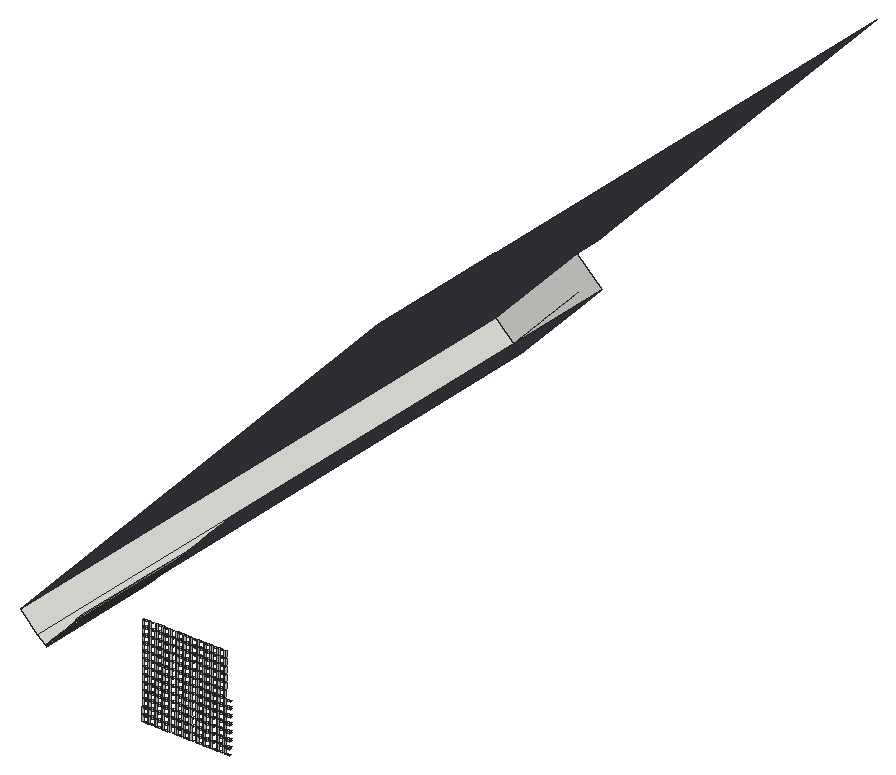
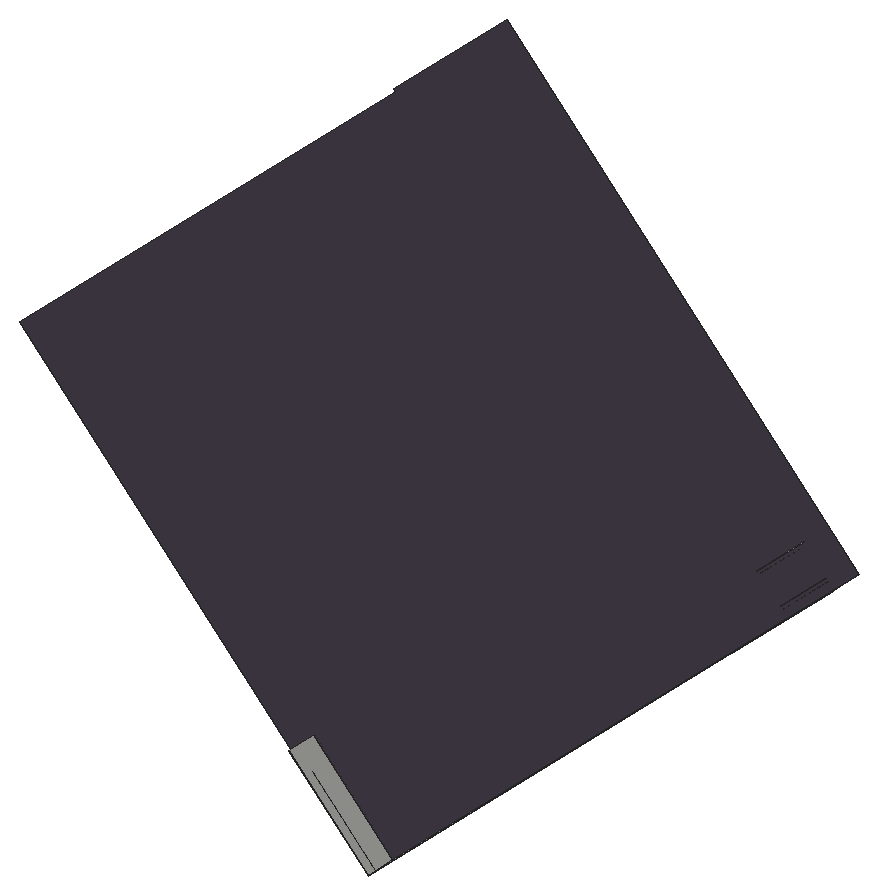
# SketchUp Ruby script. Lengths in inches.
U = 1.inch
M = Sketchup.active_model
def pt(a) = Geom::Point3d.new(a.map { |v| v * U })
def face(e, loops, mat)
  f = e.add_face(loops[0].map { |a| pt(a) })
  loops[1..].each { |l| e.add_face(l.map { |a| pt(a) }).erase! }
  f.material = f.back_material = mat if mat
  f
end
# faces: each face lists its corners as indices into pts; further lists are holes
def faces(e, pts, list, mat = nil) = list.each { |f| face(e, (f[0].is_a?(Array) ? f : [f]).map { |l| l.map { |i| pts[i] } }, mat) }
# xy, xz, yz: faces in a plane at the given z, y or x. An outline is a flat list of corners, or four numbers for a rectangle; further outlines are holes
def ring(l) = l.size == 4 ? [[l[0], l[1]], [l[2], l[1]], [l[2], l[3]], [l[0], l[3]]] : l.each_slice(2).to_a
def flat(e, list, mat, &to3) = list.each { |f| face(e, (f[0].is_a?(Array) ? f : [f]).map { |l| ring(l).map { |u, v| to3.(u, v) } }, mat) }
def xy(e, z, list, mat = nil) = flat(e, list, mat) { |x, y| [x, y, z] }
def xz(e, y, list, mat = nil) = flat(e, list, mat) { |x, z| [x, y, z] }
def yz(e, x, list, mat = nil) = flat(e, list, mat) { |y, z| [x, y, z] }
def lines(e, pts, list) = list.each { |a, b| e.add_line(pt(pts[a]), pt(pts[b])) }
# prism: a flat outline (further loops are holes) pulled along v
def prism(e, loops, v, mat = nil)
  f = face(e, loops, mat); d = Geom::Vector3d.new(v.map { |x| x * U })
  f.pushpull(f.normal.samedirection?(d) ? d.length : -d.length)
end
def box(e, o, s, mat = nil) = prism(e, [[o, [o[0] + s[0], o[1], o[2]], [o[0] + s[0], o[1] + s[1], o[2]], [o[0], o[1] + s[1], o[2]]]], [0, 0, s[2]], mat)
def at(x, y, z, deg = 0) = Geom::Transformation.translation(pt([x, y, z])) * Geom::Transformation.rotation(ORIGIN, Z_AXIS, deg.degrees)
def axes(o, x, y, z) = Geom::Transformation.new([*x, 0, *y, 0, *z, 0, *pt(o).to_a, 1])
def part(name) = M.definitions.add(name)
# library, detail: a bought-in or finely detailed component or shape, given as its bounding box
def library(name, o, s) = part(name).tap { |d| box(d.entities, o, s) }
def detail(e, o, s) = box(e.add_group.entities, o, s)
def put(e, d, t, mat = nil) = e.add_instance(d, t).tap { |i| i.material = mat if mat }
def group(e, t, mat = nil) = e.add_group.tap { |g| g.transformation = t; g.material = mat if mat }.entities
root = M.entities
M.materials.add("[Color M06]").color = [79, 71, 84]
xy(root,265.77,[[432.79,480.14,435.1,480.77],[435.7,480.14,438.02,480.77],[438.62,480.14,440.93,480.77],[441.53,480.14,443.84,480.77],[444.44,480.14,446.75,480.77],
  [447.35,480.14,449.66,480.77],[450.26,480.14,452.58,480.77],[453.18,480.14,455.49,480.77],[456.09,480.14,458.4,480.77],[459,480.14,461.3125,480.77],
  [461.91,480.14,464.22,480.77],[464.82,480.14,467.14,480.77],[467.74,480.14,470.05,480.77]])
xy(root,268.09,[[432.79,480.14,435.1,480.77],[435.7,480.14,438.02,480.77],[438.62,480.14,440.93,480.77],[441.53,480.14,443.84,480.77],[444.44,480.14,446.75,480.77],
  [447.35,480.14,449.66,480.77],[450.26,480.14,452.58,480.77],[453.18,480.14,455.49,480.77],[456.09,480.14,458.4,480.77],[459,480.14,461.3125,480.77],
  [461.91,480.14,464.22,480.77],[464.82,480.14,467.14,480.77],[467.74,480.14,470.05,480.77]])
xy(root,268.82,[[432.82,480.14,435.13,480.77],[435.73,480.14,438.05,480.77],[438.65,480.14,440.96,480.77],[441.56,480.14,443.87,480.77],[444.47,480.14,446.78,480.77],
  [447.38,480.14,449.69,480.77],[450.29,480.14,452.61,480.77],[453.21,480.14,455.52,480.77],[456.12,480.14,458.43,480.77],[459.03,480.14,461.34,480.77],
  [461.94,480.14,464.25,480.77],[464.85,480.14,467.17,480.77],[467.77,480.14,470.08,480.77]])
xy(root,271.13,[[432.82,480.14,435.13,480.77],[435.73,480.14,438.05,480.77],[438.65,480.14,440.96,480.77],[441.56,480.14,443.87,480.77],[444.47,480.14,446.78,480.77],
  [447.38,480.14,449.69,480.77],[450.29,480.14,452.61,480.77],[453.21,480.14,455.52,480.77],[456.12,480.14,458.43,480.77],[459.03,480.14,461.34,480.77],
  [461.94,480.14,464.25,480.77],[464.85,480.14,467.17,480.77],[467.77,480.14,470.08,480.77]])
xy(root,271.86,[[432.85,480.14,435.16,480.77],[435.76,480.14,438.07,480.77],[438.67,480.14,440.99,480.77],[441.59,480.14,443.9,480.77],[444.5,480.14,446.8125,480.77],
  [447.41,480.14,449.72,480.77],[450.32,480.14,452.63,480.77],[453.23,480.14,455.55,480.77],[456.15,480.14,458.46,480.77],[459.06,480.14,461.37,480.77],
  [461.97,480.14,464.28,480.77],[464.88,480.14,467.19,480.77],[467.79,480.14,470.11,480.77]])
xy(root,274.17,[[432.85,480.14,435.16,480.77],[435.76,480.14,438.07,480.77],[438.67,480.14,440.99,480.77],[441.59,480.14,443.9,480.77],[444.5,480.14,446.8125,480.77],
  [447.41,480.14,449.72,480.77],[450.32,480.14,452.63,480.77],[453.23,480.14,455.55,480.77],[456.15,480.14,458.46,480.77],[459.06,480.14,461.37,480.77],
  [461.97,480.14,464.28,480.77],[464.88,480.14,467.19,480.77],[467.79,480.14,470.11,480.77]])
xy(root,274.91,[[432.88,480.14,435.19,480.77],[435.79,480.14,438.1,480.77],[438.7,480.14,441.02,480.77],[441.62,480.14,443.93,480.77],[444.53,480.14,446.84,480.77],
  [447.4375,480.14,449.75,480.77],[450.35,480.14,452.66,480.77],[453.26,480.14,455.58,480.77],[456.18,480.14,458.49,480.77],[459.09,480.14,461.4,480.77],
  [462,480.14,464.3125,480.77],[464.91,480.14,467.22,480.77],[467.82,480.14,470.14,480.77]])
xy(root,277.22,[[432.88,480.14,435.19,480.77],[435.79,480.14,438.1,480.77],[438.7,480.14,441.02,480.77],[441.62,480.14,443.93,480.77],[444.53,480.14,446.84,480.77],
  [447.4375,480.14,449.75,480.77],[450.35,480.14,452.66,480.77],[453.26,480.14,455.58,480.77],[456.18,480.14,458.49,480.77],[459.09,480.14,461.4,480.77],
  [462,480.14,464.3125,480.77],[464.91,480.14,467.22,480.77],[467.82,480.14,470.14,480.77]])
xy(root,277.95,[[432.91,480.14,435.22,480.77],[435.82,480.14,438.13,480.77],[438.73,480.14,441.04,480.77],[441.64,480.14,443.96,480.77],[444.56,480.14,446.87,480.77],
  [447.47,480.14,449.78,480.77],[450.38,480.14,452.69,480.77],[453.29,480.14,455.6,480.77],[456.2,480.14,458.52,480.77],[459.12,480.14,461.43,480.77],
  [462.03,480.14,464.34,480.77],[464.94,480.14,467.25,480.77],[467.85,480.14,470.16,480.77]])
xy(root,280.26,[[432.91,480.14,435.22,480.77],[435.82,480.14,438.13,480.77],[438.73,480.14,441.04,480.77],[441.64,480.14,443.96,480.77],[444.56,480.14,446.87,480.77],
  [447.47,480.14,449.78,480.77],[450.38,480.14,452.69,480.77],[453.29,480.14,455.6,480.77],[456.2,480.14,458.52,480.77],[459.12,480.14,461.43,480.77],
  [462.03,480.14,464.34,480.77],[464.94,480.14,467.25,480.77],[467.85,480.14,470.16,480.77]])
xy(root,281,[[432.9375,480.14,435.25,480.77],[435.85,480.14,438.16,480.77],[438.76,480.14,441.07,480.77],[441.67,480.14,443.99,480.77],[444.59,480.14,446.9,480.77],
  [447.5,480.14,449.81,480.77],[450.41,480.14,452.72,480.77],[453.32,480.14,455.63,480.77],[456.23,480.14,458.55,480.77],[459.15,480.14,461.46,480.77],
  [462.06,480.14,464.37,480.77],[464.97,480.14,467.28,480.77],[467.88,480.14,470.19,480.77]])
xy(root,283.31,[[432.9375,480.14,435.25,480.77],[435.85,480.14,438.16,480.77],[438.76,480.14,441.07,480.77],[441.67,480.14,443.99,480.77],[444.59,480.14,446.9,480.77],
  [447.5,480.14,449.81,480.77],[450.41,480.14,452.72,480.77],[453.32,480.14,455.63,480.77],[456.23,480.14,458.55,480.77],[459.15,480.14,461.46,480.77],
  [462.06,480.14,464.37,480.77],[464.97,480.14,467.28,480.77],[467.88,480.14,470.19,480.77]])
xy(root,284.04,[[432.97,480.14,435.28,480.77],[435.88,480.14,438.19,480.77],[438.79,480.14,441.1,480.77],[441.7,480.14,444.01,480.77],[444.61,480.14,446.93,480.77],
  [447.53,480.14,449.84,480.77],[450.4375,480.14,452.75,480.77],[453.35,480.14,455.66,480.77],[456.26,480.14,458.57,480.77],[459.17,480.14,461.49,480.77],
  [462.09,480.14,464.4,480.77],[465,480.14,467.3125,480.77],[467.91,480.14,470.22,480.77]])
xy(root,286.35,[[432.97,480.14,435.28,480.77],[435.88,480.14,438.19,480.77],[438.79,480.14,441.1,480.77],[441.7,480.14,444.01,480.77],[444.61,480.14,446.93,480.77],
  [447.53,480.14,449.84,480.77],[450.4375,480.14,452.75,480.77],[453.35,480.14,455.66,480.77],[456.26,480.14,458.57,480.77],[459.17,480.14,461.49,480.77],
  [462.09,480.14,464.4,480.77],[465,480.14,467.3125,480.77],[467.91,480.14,470.22,480.77]])
xy(root,287.09,[[432.99,480.14,435.31,480.77],[435.91,480.14,438.22,480.77],[438.82,480.14,441.13,480.77],[441.73,480.14,444.04,480.77],[444.64,480.14,446.96,480.77],
  [447.56,480.14,449.87,480.77],[450.47,480.14,452.78,480.77],[453.38,480.14,455.69,480.77],[456.29,480.14,458.6,480.77],[459.2,480.14,461.52,480.77],
  [462.12,480.14,464.43,480.77],[465.03,480.14,467.34,480.77]])
xy(root,289.4,[[432.99,480.14,435.31,480.77],[435.91,480.14,438.22,480.77],[438.82,480.14,441.13,480.77],[441.73,480.14,444.04,480.77],[444.64,480.14,446.96,480.77],
  [447.56,480.14,449.87,480.77],[450.47,480.14,452.78,480.77],[453.38,480.14,455.69,480.77],[456.29,480.14,458.6,480.77],[459.2,480.14,461.52,480.77],
  [462.12,480.14,464.43,480.77],[465.03,480.14,467.34,480.77]])
xy(root,290.13,[[433.02,480.14,435.34,480.77],[435.9375,480.14,438.25,480.77],[438.85,480.14,441.16,480.77],[441.76,480.14,444.07,480.77],[444.67,480.14,446.98,480.77],
  [447.58,480.14,449.9,480.77],[450.5,480.14,452.81,480.77],[453.41,480.14,455.72,480.77],[456.32,480.14,458.63,480.77],[459.23,480.14,461.54,480.77],
  [462.14,480.14,464.46,480.77],[465.06,480.14,467.37,480.77]])
xy(root,292.44,[[433.02,480.14,435.34,480.77],[435.9375,480.14,438.25,480.77],[438.85,480.14,441.16,480.77],[441.76,480.14,444.07,480.77],[444.67,480.14,446.98,480.77],
  [447.58,480.14,449.9,480.77],[450.5,480.14,452.81,480.77],[453.41,480.14,455.72,480.77],[456.32,480.14,458.63,480.77],[459.23,480.14,461.54,480.77],
  [462.14,480.14,464.46,480.77],[465.06,480.14,467.37,480.77]])
xy(root,293.18,[[433.05,480.14,435.37,480.77],[435.96,480.14,438.28,480.77],[438.875,480.14,441.1875,480.77],[441.79,480.14,444.1,480.77],[444.7,480.14,447.01,480.77],
  [447.61,480.14,449.93,480.77],[450.53,480.14,452.84,480.77],[453.4375,480.14,455.75,480.77],[456.35,480.14,458.66,480.77],[459.26,480.14,461.57,480.77],
  [462.17,480.14,464.49,480.77],[465.09,480.14,467.4,480.77]])
xy(root,295.49,[[433.05,480.14,435.37,480.77],[435.96,480.14,438.28,480.77],[438.875,480.14,441.1875,480.77],[441.79,480.14,444.1,480.77],[444.7,480.14,447.01,480.77],
  [447.61,480.14,449.93,480.77],[450.53,480.14,452.84,480.77],[453.4375,480.14,455.75,480.77],[456.35,480.14,458.66,480.77],[459.26,480.14,461.57,480.77],
  [462.17,480.14,464.49,480.77],[465.09,480.14,467.4,480.77]])
xy(root,296.22,[[433.08,480.14,435.39,480.77],[435.99,480.14,438.31,480.77],[438.91,480.14,441.22,480.77],[441.82,480.14,444.13,480.77],[444.73,480.14,447.04,480.77],
  [447.64,480.14,449.95,480.77],[450.55,480.14,452.87,480.77],[453.47,480.14,455.78,480.77],[456.38,480.14,458.69,480.77],[459.29,480.14,461.6,480.77],
  [462.2,480.14,464.51,480.77],[465.11,480.14,467.43,480.77]])
xy(root,298.53,[[433.08,480.14,435.39,480.77],[435.99,480.14,438.31,480.77],[438.91,480.14,441.22,480.77],[441.82,480.14,444.13,480.77],[444.73,480.14,447.04,480.77],
  [447.64,480.14,449.95,480.77],[450.55,480.14,452.87,480.77],[453.47,480.14,455.78,480.77],[456.38,480.14,458.69,480.77],[459.29,480.14,461.6,480.77],
  [462.2,480.14,464.51,480.77],[465.11,480.14,467.43,480.77]])
xy(root,299.27,[[433.11,480.14,435.42,480.77],[436.02,480.14,438.34,480.77],[438.93,480.14,441.25,480.77],[441.85,480.14,444.16,480.77],[444.76,480.14,447.07,480.77],
  [447.67,480.14,449.98,480.77],[450.58,480.14,452.9,480.77],[453.5,480.14,455.81,480.77],[456.41,480.14,458.72,480.77],[459.32,480.14,461.63,480.77],
  [462.23,480.14,464.54,480.77],[465.14,480.14,467.46,480.77]])
xy(root,301.58,[[433.11,480.14,435.42,480.77],[436.02,480.14,438.34,480.77],[438.93,480.14,441.25,480.77],[441.85,480.14,444.16,480.77],[444.76,480.14,447.07,480.77],
  [447.67,480.14,449.98,480.77],[450.58,480.14,452.9,480.77],[453.5,480.14,455.81,480.77],[456.41,480.14,458.72,480.77],[459.32,480.14,461.63,480.77],
  [462.23,480.14,464.54,480.77],[465.14,480.14,467.46,480.77]])
xy(root,302.31,[[433.14,480.14,435.45,480.77],[436.05,480.14,438.36,480.77],[438.96,480.14,441.28,480.77],[441.875,480.14,444.1875,480.77],[444.79,480.14,447.1,480.77],
  [447.7,480.14,450.01,480.77],[450.61,480.14,452.92,480.77],[453.52,480.14,455.84,480.77],[456.4375,480.14,458.75,480.77],[459.35,480.14,461.66,480.77],
  [462.26,480.14,464.57,480.77],[465.17,480.14,467.48,480.77]])
xy(root,304.62,[[433.14,480.14,435.45,480.77],[436.05,480.14,438.36,480.77],[438.96,480.14,441.28,480.77],[441.875,480.14,444.1875,480.77],[444.79,480.14,447.1,480.77],
  [447.7,480.14,450.01,480.77],[450.61,480.14,452.92,480.77],[453.52,480.14,455.84,480.77],[456.4375,480.14,458.75,480.77],[459.35,480.14,461.66,480.77],
  [462.26,480.14,464.57,480.77],[465.17,480.14,467.48,480.77]])
xz(root,467.1875,[[402.58,289.13,405,291.7,404.54,292.13,402.12,289.56],[405.875,292.64,408.3,295.21,407.84,295.64,405.42,293.0625],[409.17,296.14,411.59,298.71,411.14,299.14,408.72,296.57],[412.47,299.64,414.89,302.22,414.4375,302.64,412.02,300.07],[415.77,303.15,418.19,305.72,417.74,306.15,415.32,303.58],
  [415.32,303.58,417.74,306.15,417.51,306.36,415.09,303.79]],"[Color M06]")
xz(root,521.5625,[[402.58,289.13,402.12,289.56,404.54,292.13,405,291.7],[405.875,292.64,405.42,293.0625,407.84,295.64,408.3,295.21],[409.17,296.14,408.72,296.57,411.14,299.14,411.59,298.71],[412.47,299.64,412.02,300.07,414.4375,302.64,414.89,302.22],[415.77,303.15,415.32,303.58,417.74,306.15,418.19,305.72],
  [415.32,303.58,415.09,303.79,417.51,306.36,417.74,306.15]])
xz(root,719.2,[[402.12,289.56,398.98,292.52,391.44,299.61,425.82,336.13,436.5,326.08,429.58,318.73]])
yz(root,432.79,[[480.14,265.77,480.77,268.09]])
yz(root,432.82,[[480.14,268.82,480.77,271.13]])
yz(root,432.85,[[480.14,271.86,480.77,274.17]])
yz(root,432.88,[[480.14,274.91,480.77,277.22]])
yz(root,432.91,[[480.14,277.95,480.77,280.26]])
yz(root,432.9375,[[480.14,281,480.77,283.31]])
yz(root,432.97,[[480.14,284.04,480.77,286.35]])
yz(root,432.99,[[480.14,287.09,480.77,289.4]])
yz(root,433.02,[[480.14,290.13,480.77,292.44]])
yz(root,433.05,[[480.14,293.18,480.77,295.49]])
yz(root,433.08,[[480.14,296.22,480.77,298.53]])
yz(root,433.11,[[480.14,299.27,480.77,301.58]])
yz(root,433.14,[[480.14,302.31,480.77,304.62]])
yz(root,435.1,[[480.14,265.77,480.77,268.09]])
yz(root,435.13,[[480.14,268.82,480.77,271.13]])
yz(root,435.16,[[480.14,271.86,480.77,274.17]])
yz(root,435.19,[[480.14,274.91,480.77,277.22]])
yz(root,435.22,[[480.14,277.95,480.77,280.26]])
yz(root,435.25,[[480.14,281,480.77,283.31]])
yz(root,435.28,[[480.14,284.04,480.77,286.35]])
yz(root,435.31,[[480.14,287.09,480.77,289.4]])
yz(root,435.34,[[480.14,290.13,480.77,292.44]])
yz(root,435.37,[[480.14,293.18,480.77,295.49]])
yz(root,435.39,[[480.14,296.22,480.77,298.53]])
yz(root,435.42,[[480.14,299.27,480.77,301.58]])
yz(root,435.45,[[480.14,302.31,480.77,304.62]])
yz(root,435.7,[[480.14,265.77,480.77,268.09]])
yz(root,435.73,[[480.14,268.82,480.77,271.13]])
yz(root,435.76,[[480.14,271.86,480.77,274.17]])
yz(root,435.79,[[480.14,274.91,480.77,277.22]])
yz(root,435.82,[[480.14,277.95,480.77,280.26]])
yz(root,435.85,[[480.14,281,480.77,283.31]])
yz(root,435.88,[[480.14,284.04,480.77,286.35]])
yz(root,435.91,[[480.14,287.09,480.77,289.4]])
yz(root,435.9375,[[480.14,290.13,480.77,292.44]])
yz(root,435.96,[[480.14,293.18,480.77,295.49]])
yz(root,435.99,[[480.14,296.22,480.77,298.53]])
yz(root,436.02,[[480.14,299.27,480.77,301.58]])
yz(root,436.05,[[480.14,302.31,480.77,304.62]])
yz(root,438.02,[[480.14,265.77,480.77,268.09]])
yz(root,438.05,[[480.14,268.82,480.77,271.13]])
yz(root,438.07,[[480.14,271.86,480.77,274.17]])
yz(root,438.1,[[480.14,274.91,480.77,277.22]])
yz(root,438.13,[[480.14,277.95,480.77,280.26]])
yz(root,438.16,[[480.14,281,480.77,283.31]])
yz(root,438.19,[[480.14,284.04,480.77,286.35]])
yz(root,438.22,[[480.14,287.09,480.77,289.4]])
yz(root,438.25,[[480.14,290.13,480.77,292.44]])
yz(root,438.28,[[480.14,293.18,480.77,295.49]])
yz(root,438.31,[[480.14,296.22,480.77,298.53]])
yz(root,438.34,[[480.14,299.27,480.77,301.58]])
yz(root,438.36,[[480.14,302.31,480.77,304.62]])
yz(root,438.62,[[480.14,265.77,480.77,268.09]])
yz(root,438.65,[[480.14,268.82,480.77,271.13]])
yz(root,438.67,[[480.14,271.86,480.77,274.17]])
yz(root,438.7,[[480.14,274.91,480.77,277.22]])
yz(root,438.73,[[480.14,277.95,480.77,280.26]])
yz(root,438.76,[[480.14,281,480.77,283.31]])
yz(root,438.79,[[480.14,284.04,480.77,286.35]])
yz(root,438.82,[[480.14,287.09,480.77,289.4]])
yz(root,438.85,[[480.14,290.13,480.77,292.44]])
yz(root,438.875,[[480.14,293.18,480.77,295.49]])
yz(root,438.91,[[480.14,296.22,480.77,298.53]])
yz(root,438.93,[[480.14,299.27,480.77,301.58]])
yz(root,438.96,[[480.14,302.31,480.77,304.62]])
yz(root,440.93,[[480.14,265.77,480.77,268.09]])
yz(root,440.96,[[480.14,268.82,480.77,271.13]])
yz(root,440.99,[[480.14,271.86,480.77,274.17]])
yz(root,441.02,[[480.14,274.91,480.77,277.22]])
yz(root,441.04,[[480.14,277.95,480.77,280.26]])
yz(root,441.07,[[480.14,281,480.77,283.31]])
yz(root,441.1,[[480.14,284.04,480.77,286.35]])
yz(root,441.13,[[480.14,287.09,480.77,289.4]])
yz(root,441.16,[[480.14,290.13,480.77,292.44]])
yz(root,441.1875,[[480.14,293.18,480.77,295.49]])
yz(root,441.22,[[480.14,296.22,480.77,298.53]])
yz(root,441.25,[[480.14,299.27,480.77,301.58]])
yz(root,441.28,[[480.14,302.31,480.77,304.62]])
yz(root,441.53,[[480.14,265.77,480.77,268.09]])
yz(root,441.56,[[480.14,268.82,480.77,271.13]])
yz(root,441.59,[[480.14,271.86,480.77,274.17]])
yz(root,441.62,[[480.14,274.91,480.77,277.22]])
yz(root,441.64,[[480.14,277.95,480.77,280.26]])
yz(root,441.67,[[480.14,281,480.77,283.31]])
yz(root,441.7,[[480.14,284.04,480.77,286.35]])
yz(root,441.73,[[480.14,287.09,480.77,289.4]])
yz(root,441.76,[[480.14,290.13,480.77,292.44]])
yz(root,441.79,[[480.14,293.18,480.77,295.49]])
yz(root,441.82,[[480.14,296.22,480.77,298.53]])
yz(root,441.85,[[480.14,299.27,480.77,301.58]])
yz(root,441.875,[[480.14,302.31,480.77,304.62]])
yz(root,443.84,[[480.14,265.77,480.77,268.09]])
yz(root,443.87,[[480.14,268.82,480.77,271.13]])
yz(root,443.9,[[480.14,271.86,480.77,274.17]])
yz(root,443.93,[[480.14,274.91,480.77,277.22]])
yz(root,443.96,[[480.14,277.95,480.77,280.26]])
yz(root,443.99,[[480.14,281,480.77,283.31]])
yz(root,444.01,[[480.14,284.04,480.77,286.35]])
yz(root,444.04,[[480.14,287.09,480.77,289.4]])
yz(root,444.07,[[480.14,290.13,480.77,292.44]])
yz(root,444.1,[[480.14,293.18,480.77,295.49]])
yz(root,444.13,[[480.14,296.22,480.77,298.53]])
yz(root,444.16,[[480.14,299.27,480.77,301.58]])
yz(root,444.1875,[[480.14,302.31,480.77,304.62]])
yz(root,444.44,[[480.14,265.77,480.77,268.09]])
yz(root,444.47,[[480.14,268.82,480.77,271.13]])
yz(root,444.5,[[480.14,271.86,480.77,274.17]])
yz(root,444.53,[[480.14,274.91,480.77,277.22]])
yz(root,444.56,[[480.14,277.95,480.77,280.26]])
yz(root,444.59,[[480.14,281,480.77,283.31]])
yz(root,444.61,[[480.14,284.04,480.77,286.35]])
yz(root,444.64,[[480.14,287.09,480.77,289.4]])
yz(root,444.67,[[480.14,290.13,480.77,292.44]])
yz(root,444.7,[[480.14,293.18,480.77,295.49]])
yz(root,444.73,[[480.14,296.22,480.77,298.53]])
yz(root,444.76,[[480.14,299.27,480.77,301.58]])
yz(root,444.79,[[480.14,302.31,480.77,304.62]])
yz(root,446.75,[[480.14,265.77,480.77,268.09]])
yz(root,446.78,[[480.14,268.82,480.77,271.13]])
yz(root,446.8125,[[480.14,271.86,480.77,274.17]])
yz(root,446.84,[[480.14,274.91,480.77,277.22]])
yz(root,446.87,[[480.14,277.95,480.77,280.26]])
yz(root,446.9,[[480.14,281,480.77,283.31]])
yz(root,446.93,[[480.14,284.04,480.77,286.35]])
yz(root,446.96,[[480.14,287.09,480.77,289.4]])
yz(root,446.98,[[480.14,290.13,480.77,292.44]])
yz(root,447.01,[[480.14,293.18,480.77,295.49]])
yz(root,447.04,[[480.14,296.22,480.77,298.53]])
yz(root,447.07,[[480.14,299.27,480.77,301.58]])
yz(root,447.1,[[480.14,302.31,480.77,304.62]])
yz(root,447.35,[[480.14,265.77,480.77,268.09]])
yz(root,447.38,[[480.14,268.82,480.77,271.13]])
yz(root,447.41,[[480.14,271.86,480.77,274.17]])
yz(root,447.4375,[[480.14,274.91,480.77,277.22]])
yz(root,447.47,[[480.14,277.95,480.77,280.26]])
yz(root,447.5,[[480.14,281,480.77,283.31]])
yz(root,447.53,[[480.14,284.04,480.77,286.35]])
yz(root,447.56,[[480.14,287.09,480.77,289.4]])
yz(root,447.58,[[480.14,290.13,480.77,292.44]])
yz(root,447.61,[[480.14,293.18,480.77,295.49]])
yz(root,447.64,[[480.14,296.22,480.77,298.53]])
yz(root,447.67,[[480.14,299.27,480.77,301.58]])
yz(root,447.7,[[480.14,302.31,480.77,304.62]])
yz(root,449.66,[[480.14,265.77,480.77,268.09]])
yz(root,449.69,[[480.14,268.82,480.77,271.13]])
yz(root,449.72,[[480.14,271.86,480.77,274.17]])
yz(root,449.75,[[480.14,274.91,480.77,277.22]])
yz(root,449.78,[[480.14,277.95,480.77,280.26]])
yz(root,449.81,[[480.14,281,480.77,283.31]])
yz(root,449.84,[[480.14,284.04,480.77,286.35]])
yz(root,449.87,[[480.14,287.09,480.77,289.4]])
yz(root,449.9,[[480.14,290.13,480.77,292.44]])
yz(root,449.93,[[480.14,293.18,480.77,295.49]])
yz(root,449.95,[[480.14,296.22,480.77,298.53]])
yz(root,449.98,[[480.14,299.27,480.77,301.58]])
yz(root,450.01,[[480.14,302.31,480.77,304.62]])
yz(root,450.26,[[480.14,265.77,480.77,268.09]])
yz(root,450.29,[[480.14,268.82,480.77,271.13]])
yz(root,450.32,[[480.14,271.86,480.77,274.17]])
yz(root,450.35,[[480.14,274.91,480.77,277.22]])
yz(root,450.38,[[480.14,277.95,480.77,280.26]])
yz(root,450.41,[[480.14,281,480.77,283.31]])
yz(root,450.4375,[[480.14,284.04,480.77,286.35]])
yz(root,450.47,[[480.14,287.09,480.77,289.4]])
yz(root,450.5,[[480.14,290.13,480.77,292.44]])
yz(root,450.53,[[480.14,293.18,480.77,295.49]])
yz(root,450.55,[[480.14,296.22,480.77,298.53]])
yz(root,450.58,[[480.14,299.27,480.77,301.58]])
yz(root,450.61,[[480.14,302.31,480.77,304.62]])
yz(root,452.58,[[480.14,265.77,480.77,268.09]])
yz(root,452.61,[[480.14,268.82,480.77,271.13]])
yz(root,452.63,[[480.14,271.86,480.77,274.17]])
yz(root,452.66,[[480.14,274.91,480.77,277.22]])
yz(root,452.69,[[480.14,277.95,480.77,280.26]])
yz(root,452.72,[[480.14,281,480.77,283.31]])
yz(root,452.75,[[480.14,284.04,480.77,286.35]])
yz(root,452.78,[[480.14,287.09,480.77,289.4]])
yz(root,452.81,[[480.14,290.13,480.77,292.44]])
yz(root,452.84,[[480.14,293.18,480.77,295.49]])
yz(root,452.87,[[480.14,296.22,480.77,298.53]])
yz(root,452.9,[[480.14,299.27,480.77,301.58]])
yz(root,452.92,[[480.14,302.31,480.77,304.62]])
yz(root,453.18,[[480.14,265.77,480.77,268.09]])
yz(root,453.21,[[480.14,268.82,480.77,271.13]])
yz(root,453.23,[[480.14,271.86,480.77,274.17]])
yz(root,453.26,[[480.14,274.91,480.77,277.22]])
yz(root,453.29,[[480.14,277.95,480.77,280.26]])
yz(root,453.32,[[480.14,281,480.77,283.31]])
yz(root,453.35,[[480.14,284.04,480.77,286.35]])
yz(root,453.38,[[480.14,287.09,480.77,289.4]])
yz(root,453.41,[[480.14,290.13,480.77,292.44]])
yz(root,453.4375,[[480.14,293.18,480.77,295.49]])
yz(root,453.47,[[480.14,296.22,480.77,298.53]])
yz(root,453.5,[[480.14,299.27,480.77,301.58]])
yz(root,453.52,[[480.14,302.31,480.77,304.62]])
yz(root,455.49,[[480.14,265.77,480.77,268.09]])
yz(root,455.52,[[480.14,268.82,480.77,271.13]])
yz(root,455.55,[[480.14,271.86,480.77,274.17]])
yz(root,455.58,[[480.14,274.91,480.77,277.22]])
yz(root,455.6,[[480.14,277.95,480.77,280.26]])
yz(root,455.63,[[480.14,281,480.77,283.31]])
yz(root,455.66,[[480.14,284.04,480.77,286.35]])
yz(root,455.69,[[480.14,287.09,480.77,289.4]])
yz(root,455.72,[[480.14,290.13,480.77,292.44]])
yz(root,455.75,[[480.14,293.18,480.77,295.49]])
yz(root,455.78,[[480.14,296.22,480.77,298.53]])
yz(root,455.81,[[480.14,299.27,480.77,301.58]])
yz(root,455.84,[[480.14,302.31,480.77,304.62]])
yz(root,456.09,[[480.14,265.77,480.77,268.09]])
yz(root,456.12,[[480.14,268.82,480.77,271.13]])
yz(root,456.15,[[480.14,271.86,480.77,274.17]])
yz(root,456.18,[[480.14,274.91,480.77,277.22]])
yz(root,456.2,[[480.14,277.95,480.77,280.26]])
yz(root,456.23,[[480.14,281,480.77,283.31]])
yz(root,456.26,[[480.14,284.04,480.77,286.35]])
yz(root,456.29,[[480.14,287.09,480.77,289.4]])
yz(root,456.32,[[480.14,290.13,480.77,292.44]])
yz(root,456.35,[[480.14,293.18,480.77,295.49]])
yz(root,456.38,[[480.14,296.22,480.77,298.53]])
yz(root,456.41,[[480.14,299.27,480.77,301.58]])
yz(root,456.4375,[[480.14,302.31,480.77,304.62]])
yz(root,458.4,[[480.14,265.77,480.77,268.09]])
yz(root,458.43,[[480.14,268.82,480.77,271.13]])
yz(root,458.46,[[480.14,271.86,480.77,274.17]])
yz(root,458.49,[[480.14,274.91,480.77,277.22]])
yz(root,458.52,[[480.14,277.95,480.77,280.26]])
yz(root,458.55,[[480.14,281,480.77,283.31]])
yz(root,458.57,[[480.14,284.04,480.77,286.35]])
yz(root,458.6,[[480.14,287.09,480.77,289.4]])
yz(root,458.63,[[480.14,290.13,480.77,292.44]])
yz(root,458.66,[[480.14,293.18,480.77,295.49]])
yz(root,458.69,[[480.14,296.22,480.77,298.53]])
yz(root,458.72,[[480.14,299.27,480.77,301.58]])
yz(root,458.75,[[480.14,302.31,480.77,304.62]])
yz(root,459,[[480.14,265.77,480.77,268.09]])
yz(root,459.03,[[480.14,268.82,480.77,271.13]])
yz(root,459.06,[[480.14,271.86,480.77,274.17]])
yz(root,459.09,[[480.14,274.91,480.77,277.22]])
yz(root,459.12,[[480.14,277.95,480.77,280.26]])
yz(root,459.15,[[480.14,281,480.77,283.31]])
yz(root,459.17,[[480.14,284.04,480.77,286.35]])
yz(root,459.2,[[480.14,287.09,480.77,289.4]])
yz(root,459.23,[[480.14,290.13,480.77,292.44]])
yz(root,459.26,[[480.14,293.18,480.77,295.49]])
yz(root,459.29,[[480.14,296.22,480.77,298.53]])
yz(root,459.32,[[480.14,299.27,480.77,301.58]])
yz(root,459.35,[[480.14,302.31,480.77,304.62]])
yz(root,461.3125,[[480.14,265.77,480.77,268.09]])
yz(root,461.34,[[480.14,268.82,480.77,271.13]])
yz(root,461.37,[[480.14,271.86,480.77,274.17]])
yz(root,461.4,[[480.14,274.91,480.77,277.22]])
yz(root,461.43,[[480.14,277.95,480.77,280.26]])
yz(root,461.46,[[480.14,281,480.77,283.31]])
yz(root,461.49,[[480.14,284.04,480.77,286.35]])
yz(root,461.52,[[480.14,287.09,480.77,289.4]])
yz(root,461.54,[[480.14,290.13,480.77,292.44]])
yz(root,461.57,[[480.14,293.18,480.77,295.49]])
yz(root,461.6,[[480.14,296.22,480.77,298.53]])
yz(root,461.63,[[480.14,299.27,480.77,301.58]])
yz(root,461.66,[[480.14,302.31,480.77,304.62]])
yz(root,461.91,[[480.14,265.77,480.77,268.09]])
yz(root,461.94,[[480.14,268.82,480.77,271.13]])
yz(root,461.97,[[480.14,271.86,480.77,274.17]])
yz(root,462,[[480.14,274.91,480.77,277.22]])
yz(root,462.03,[[480.14,277.95,480.77,280.26]])
yz(root,462.06,[[480.14,281,480.77,283.31]])
yz(root,462.09,[[480.14,284.04,480.77,286.35]])
yz(root,462.12,[[480.14,287.09,480.77,289.4]])
yz(root,462.14,[[480.14,290.13,480.77,292.44]])
yz(root,462.17,[[480.14,293.18,480.77,295.49]])
yz(root,462.2,[[480.14,296.22,480.77,298.53]])
yz(root,462.23,[[480.14,299.27,480.77,301.58]])
yz(root,462.26,[[480.14,302.31,480.77,304.62]])
yz(root,464.22,[[480.14,265.77,480.77,268.09]])
yz(root,464.25,[[480.14,268.82,480.77,271.13]])
yz(root,464.28,[[480.14,271.86,480.77,274.17]])
yz(root,464.3125,[[480.14,274.91,480.77,277.22]])
yz(root,464.34,[[480.14,277.95,480.77,280.26]])
yz(root,464.37,[[480.14,281,480.77,283.31]])
yz(root,464.4,[[480.14,284.04,480.77,286.35]])
yz(root,464.43,[[480.14,287.09,480.77,289.4]])
yz(root,464.46,[[480.14,290.13,480.77,292.44]])
yz(root,464.49,[[480.14,293.18,480.77,295.49]])
yz(root,464.51,[[480.14,296.22,480.77,298.53]])
yz(root,464.54,[[480.14,299.27,480.77,301.58]])
yz(root,464.57,[[480.14,302.31,480.77,304.62]])
yz(root,464.82,[[480.14,265.77,480.77,268.09]])
yz(root,464.85,[[480.14,268.82,480.77,271.13]])
yz(root,464.88,[[480.14,271.86,480.77,274.17]])
yz(root,464.91,[[480.14,274.91,480.77,277.22]])
yz(root,464.94,[[480.14,277.95,480.77,280.26]])
yz(root,464.97,[[480.14,281,480.77,283.31]])
yz(root,465,[[480.14,284.04,480.77,286.35]])
yz(root,465.03,[[480.14,287.09,480.77,289.4]])
yz(root,465.06,[[480.14,290.13,480.77,292.44]])
yz(root,465.09,[[480.14,293.18,480.77,295.49]])
yz(root,465.11,[[480.14,296.22,480.77,298.53]])
yz(root,465.14,[[480.14,299.27,480.77,301.58]])
yz(root,465.17,[[480.14,302.31,480.77,304.62]])
yz(root,467.14,[[480.14,265.77,480.77,268.09]])
yz(root,467.17,[[480.14,268.82,480.77,271.13]])
yz(root,467.19,[[480.14,271.86,480.77,274.17]])
yz(root,467.22,[[480.14,274.91,480.77,277.22]])
yz(root,467.25,[[480.14,277.95,480.77,280.26]])
yz(root,467.28,[[480.14,281,480.77,283.31]])
yz(root,467.3125,[[480.14,284.04,480.77,286.35]])
yz(root,467.34,[[480.14,287.09,480.77,289.4]])
yz(root,467.37,[[480.14,290.13,480.77,292.44]])
yz(root,467.4,[[480.14,293.18,480.77,295.49]])
yz(root,467.43,[[480.14,296.22,480.77,298.53]])
yz(root,467.46,[[480.14,299.27,480.77,301.58]])
yz(root,467.48,[[480.14,302.31,480.77,304.62]])
yz(root,467.74,[[480.14,265.77,480.77,268.09]])
yz(root,467.77,[[480.14,268.82,480.77,271.13]])
yz(root,467.79,[[480.14,271.86,480.77,274.17]])
yz(root,467.82,[[480.14,274.91,480.77,277.22]])
yz(root,467.85,[[480.14,277.95,480.77,280.26]])
yz(root,467.88,[[480.14,281,480.77,283.31]])
yz(root,467.91,[[480.14,284.04,480.77,286.35]])
yz(root,467.9375,[[480.14,287.09,480.77,289.4]])
yz(root,467.97,[[480.14,290.13,480.77,292.44]])
yz(root,468,[[480.14,293.18,480.77,295.49]])
yz(root,468.03,[[480.14,296.22,480.77,298.53]])
yz(root,468.06,[[480.14,299.27,480.77,301.58]])
yz(root,468.08,[[480.14,302.31,480.77,304.62]])
p = [[402.12,467.1875,289.56],[402.12,521.5625,289.56],[402.58,521.5625,289.13],[402.58,467.1875,289.13],[405,521.5625,291.7],[405,467.1875,291.7],
  [398.98,467.1875,292.52],[398.98,528.48,292.52],[398.98,719.2,292.52],[402.12,719.2,289.56],[404.54,521.5625,292.13],[404.54,467.1875,292.13],
  [436.5,719.2,326.08],[436.5,528.48,326.08],[436.5,521.5625,326.08],[435.11,521.5625,324.6],[434.23,521.5625,323.67],[431.81,521.5625,321.1],
  [430.93,521.5625,320.17],[429.58,521.5625,318.73],[428.51,521.5625,317.59],[427.63,521.5625,316.66],[425.21,521.5625,314.09],[424.33,521.5625,313.16],
  [421.91,521.5625,310.59],[421.04,521.5625,309.65],[418.61,521.5625,307.08],[417.74,521.5625,306.15],[415.32,521.5625,303.58],[414.4375,521.5625,302.64],
  [412.02,521.5625,300.07],[411.14,521.5625,299.14],[408.72,521.5625,296.57],[407.84,521.5625,295.64],[405.42,521.5625,293.0625],[429.58,719.2,318.73],
  [405.42,467.1875,293.0625],[391.44,467.1875,299.61],[391.44,719.2,299.61],[405.875,521.5625,292.64],[405.875,467.1875,292.64],[408.3,521.5625,295.21],
  [408.3,467.1875,295.21],[407.84,467.1875,295.64],[408.72,467.1875,296.57],[409.17,521.5625,296.14],[409.17,467.1875,296.14],[411.59,521.5625,298.71],
  [411.59,467.1875,298.71],[411.14,467.1875,299.14],[412.02,467.1875,300.07],[543.65,467.1875,461.31],[543.65,528.48,461.31],[542.88,528.48,460.49],
  [542.88,731.75,460.49],[446.875,731.75,358.5],[446.15,731.75,357.73],[429.58,731.75,340.125],[425.82,731.75,336.13],[425.82,719.2,336.13],
  [412.47,521.5625,299.64],[412.47,467.1875,299.64],[414.89,521.5625,302.22],[414.89,467.1875,302.22],[414.4375,467.1875,302.64],[415.32,467.1875,303.58],
  [415.77,521.5625,303.15],[415.77,467.1875,303.15],[418.19,521.5625,305.72],[418.19,467.1875,305.72],[415.09,467.1875,303.79],[415.09,521.5625,303.79],
  [417.74,467.1875,306.15],[417.51,521.5625,306.36],[417.51,467.1875,306.36],[426.44,719.2,321.6875]]
faces(root,p,[[0,1,2,3],[0,6,7,8,9,1],[10,1,0,11],[10,11,5,4],[6,37,38,8,7],[36,34,39,40],[33,34,36,43],[33,43,42,41],
  [44,32,45,46],[31,32,44,49],[31,49,48,47],[50,30,60,61],[29,30,50,64],[29,64,63,62],[28,65,70,71],[27,28,65,72],
  [73,71,70,74]])
faces(root,p,[[2,4,5,3],[12,13,14,15,16,17,18,19,20,21,22,23,24,25,26,27,28,29,30,31,32,33,34,10,1,9,35],[10,34,36,11],[39,41,42,40],[33,32,44,43],[45,47,48,46],[31,30,50,49],[38,37,51,52,53,54,55,56,57,58,59],
  [60,62,63,61],[29,28,65,64],[65,28,66,67],[66,68,69,67]],"[Color M06]")
lines(root,p,[[75,8]])
